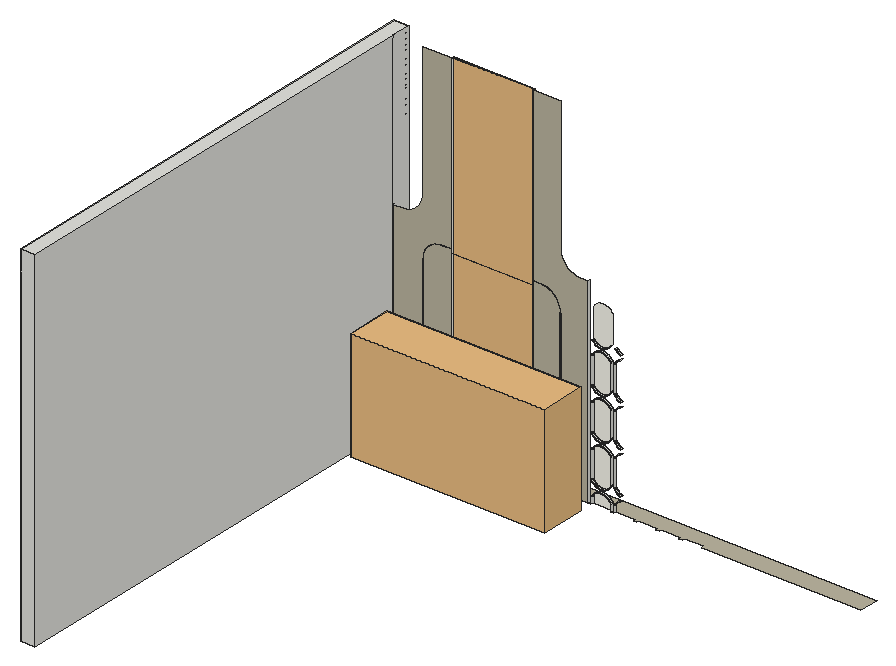
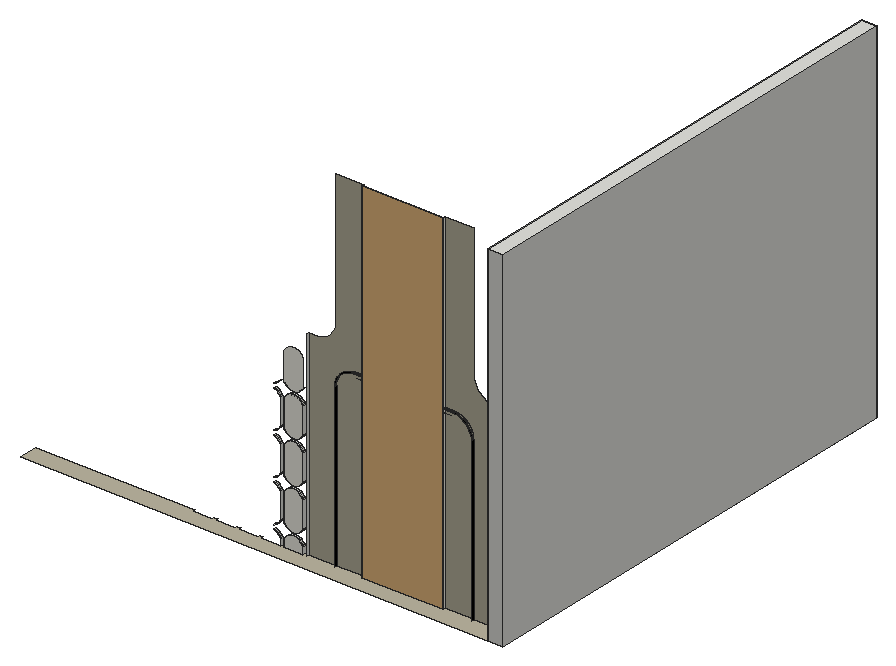
# SketchUp Ruby script. Lengths in inches.
U = 1.inch
M = Sketchup.active_model
def pt(a) = Geom::Point3d.new(a.map { |v| v * U })
def face(e, loops, mat)
  f = e.add_face(loops[0].map { |a| pt(a) })
  loops[1..].each { |l| e.add_face(l.map { |a| pt(a) }).erase! }
  f.material = f.back_material = mat if mat
  f
end
# faces: each face lists its corners as indices into pts; further lists are holes
def faces(e, pts, list, mat = nil) = list.each { |f| face(e, (f[0].is_a?(Array) ? f : [f]).map { |l| l.map { |i| pts[i] } }, mat) }
# xy, xz, yz: faces in a plane at the given z, y or x. An outline is a flat list of corners, or four numbers for a rectangle; further outlines are holes
def ring(l) = l.size == 4 ? [[l[0], l[1]], [l[2], l[1]], [l[2], l[3]], [l[0], l[3]]] : l.each_slice(2).to_a
def flat(e, list, mat, &to3) = list.each { |f| face(e, (f[0].is_a?(Array) ? f : [f]).map { |l| ring(l).map { |u, v| to3.(u, v) } }, mat) }
def xy(e, z, list, mat = nil) = flat(e, list, mat) { |x, y| [x, y, z] }
def xz(e, y, list, mat = nil) = flat(e, list, mat) { |x, z| [x, y, z] }
def yz(e, x, list, mat = nil) = flat(e, list, mat) { |y, z| [x, y, z] }
def lines(e, pts, list) = list.each { |a, b| e.add_line(pt(pts[a]), pt(pts[b])) }
# prism: a flat outline (further loops are holes) pulled along v
def prism(e, loops, v, mat = nil)
  f = face(e, loops, mat); d = Geom::Vector3d.new(v.map { |x| x * U })
  f.pushpull(f.normal.samedirection?(d) ? d.length : -d.length)
end
def box(e, o, s, mat = nil) = prism(e, [[o, [o[0] + s[0], o[1], o[2]], [o[0] + s[0], o[1] + s[1], o[2]], [o[0], o[1] + s[1], o[2]]]], [0, 0, s[2]], mat)
def at(x, y, z, deg = 0) = Geom::Transformation.translation(pt([x, y, z])) * Geom::Transformation.rotation(ORIGIN, Z_AXIS, deg.degrees)
def axes(o, x, y, z) = Geom::Transformation.new([*x, 0, *y, 0, *z, 0, *pt(o).to_a, 1])
def part(name) = M.definitions.add(name)
# library, detail: a bought-in or finely detailed component or shape, given as its bounding box
def library(name, o, s) = part(name).tap { |d| box(d.entities, o, s) }
def detail(e, o, s) = box(e.add_group.entities, o, s)
def put(e, d, t, mat = nil) = e.add_instance(d, t).tap { |i| i.material = mat if mat }
def group(e, t, mat = nil) = e.add_group.tap { |g| g.transformation = t; g.material = mat if mat }.entities
root = M.entities
M.materials.add("Tafisa-Gardenia-or-Gardenia-PM775-4K").color = [246, 245, 235]
M.materials.add("Uniboard-L19-Putty-4K").color = [187, 181, 160]
M.materials.add("[Color M09]").color = [0, 0, 0]
c1 = part("Group196\#1")
p = [[0,0,0],[0,0,-16.77],[-0.04,0,-16.77],[0.28,-54,0],[-0.28,-54,0],[0.28,54,0],
  [0.28,0,0],[-0.28,54,0],[0.04,0,-16.77],[-0.28,0,0],[0,0,-27.14]]
lines(c1.entities,p,[[0,1],[1,2],[3,4],[5,6],[7,5],[1,8],[9,0],[0,6],[8,10],[4,9],[6,3],[2,10],
  [9,7]])
c2 = part("Rectangle Light\#1")
put(c2.entities,c1,at(0,0,0))
c3 = library("Group3\#1",[-12.5,-54,0],[24.96,108,0.24])
c4 = library("Group\#6",[0,0,0],[59.84,14,34])
c5 = part("Group194\#1")
p = [[0,0,0],[0,0,-16.77],[-0.04,0,-16.77],[0.28,-54,0],[-0.28,-54,0],[0.28,54,0],
  [0.28,0,0],[-0.28,54,0],[0.04,0,-16.77],[-0.28,0,0],[0,0,-27.14]]
lines(c5.entities,p,[[0,1],[1,2],[3,4],[5,6],[7,5],[1,8],[9,0],[0,6],[8,10],[4,9],[6,3],[2,10],
  [9,7]])
c6 = part("Rectangle Light")
put(c6.entities,c5,at(0,0,0))
xy(root,6,[[4.5,138,4.5,144,148.5,144,148.5,138,100.62,138,100.62,138.71,100.5,138.71,100.5,138,99.5,138,99.5,138.79,93.5625,138.79,93.5625,138,92.5625,138,92.5625,138.79,86.5,138.79,86.5,138,85.5,138,85.5,138.79,79.5,138.79,79.5,138,78.5,138,78.5,138.79,72.5,138.79,72.5,138,71.5,138,71.5,138.79,65.5,138.79,65.5,138,64.5,138,64.5,138.71,64.38,138.71,64.38,138,56,138,56,138.71,55.76,138.71,55.76,138,47.5,138,47.5,138.79,22.5,138.79,22.5,138,13.74,138,13.74,138.71,13.5,138.71,13.5,138]],"Uniboard-L19-Putty-4K")
xz(root,138,[[4.5,6,13.5,6,13.5,55.5,13.55,56.28,13.7,57.05,13.96,57.8,14.3,58.5,14.74,59.15,15.26,59.74,15.85,60.26,16.5,60.7,17.2,61.04,17.95,61.3,18.72,61.45,19.5,61.5,22.5,61.5,22.5,114,13.5,114,13.5,73.3125,13.45,72.53,13.3,71.76,13.04,71.02,12.7,70.3125,12.26,69.66,11.74,69.07,11.15,68.55,10.5,68.12,9.8,67.77,9.05,67.52,8.28,67.36,7.5,67.3125,4.5,67.3125],[13.74,6,22.5,6,22.5,61.26,19.5,61.26,18.75,61.21,18.01,61.07,17.29,60.83,16.62,60.49,15.99,60.07,15.42,59.58,14.93,59.01,14.51,58.38,14.17,57.71,13.93,56.99,13.79,56.25,13.74,55.5],[47.5,6,55.76,6,55.76,55.5,55.71,56.25,55.57,56.99,55.33,57.71,54.99,58.38,54.57,59.01,54.08,59.58,53.51,60.07,52.88,60.49,52.21,60.83,51.49,61.07,50.75,61.21,50,61.26,47.5,61.26],[56,6,64.38,6,64.38,67.3125,62,67.3125,61.22,67.36,60.45,67.52,59.7,67.77,59,68.12,58.35,68.55,57.76,69.07,57.24,69.66,56.8,70.3125,56.46,71.02,56.2,71.76,56.05,72.53,56,73.3125,56,114,47.5,114,47.5,61.5,50,61.5,50.78,61.45,51.55,61.3,52.3,61.04,53,60.7,53.65,60.26,54.24,59.74,54.76,59.15,55.2,58.5,55.54,57.8,55.8,57.05,55.95,56.28,56,55.5]],"Uniboard-L19-Putty-4K")
xz(root,138.71,[[64.38,6,64.5,67.3125]])
xz(root,138.71,[[13.5,6,13.74,6,13.74,55.5,13.79,56.25,13.93,56.99,14.17,57.71,14.51,58.38,14.93,59.01,15.42,59.58,15.99,60.07,16.62,60.49,17.29,60.83,18.01,61.07,18.75,61.21,19.5,61.26,22.5,61.26,22.5,61.5,19.5,61.5,18.72,61.45,17.95,61.3,17.2,61.04,16.5,60.7,15.85,60.26,15.26,59.74,14.74,59.15,14.3,58.5,13.96,57.8,13.7,57.05,13.55,56.28,13.5,55.5],[55.76,6,56,6,56,55.5,55.95,56.28,55.8,57.05,55.54,57.8,55.2,58.5,54.76,59.15,54.24,59.74,53.65,60.26,53,60.7,52.3,61.04,51.55,61.3,50.78,61.45,50,61.5,47.5,61.5,47.5,61.26,50,61.26,50.75,61.21,51.49,61.07,52.21,60.83,52.88,60.49,53.51,60.07,54.08,59.58,54.57,59.01,54.99,58.38,55.33,57.71,55.57,56.99,55.71,56.25,55.76,55.5]],"[Color M09]")
xz(root,138.79,[[65.5,6,71.5,6,71.5,8,71.36,8.29,71.2,8.56,71.01,8.82,70.79,9.05,70.56,9.26,70.3,9.45,70.03,9.62,69.74,9.75,69.44,9.86,69.13,9.9375,68.82,9.98,68.5,10,68.18,9.98,67.87,9.9375,67.56,9.86,67.26,9.75,66.97,9.62,66.7,9.45,66.44,9.26,66.21,9.05,65.99,8.82,65.8,8.56,65.64,8.29,65.5,8],[68.5,11,68.82,11.02,69.13,11.0625,69.44,11.14,69.74,11.25,70.03,11.38,70.3,11.55,70.56,11.74,70.79,11.95,71.01,12.18,71.2,12.44,71.36,12.71,71.5,13,71.5,21,71.36,21.29,71.2,21.56,71.01,21.82,70.79,22.05,70.56,22.26,70.3,22.45,70.03,22.62,69.74,22.75,69.44,22.86,69.13,22.9375,68.82,22.98,68.5,23,68.18,22.98,67.87,22.9375,67.56,22.86,67.26,22.75,66.97,22.62,66.7,22.45,66.44,22.26,66.21,22.05,65.99,21.82,65.8,21.56,65.64,21.29,65.5,21,65.5,13,65.64,12.71,65.8,12.44,65.99,12.18,66.21,11.95,66.44,11.74,66.7,11.55,66.97,11.38,67.26,11.25,67.56,11.14,67.87,11.0625,68.18,11.02],[68.5,24,68.82,24.02,69.13,24.0625,69.44,24.14,69.74,24.25,70.03,24.38,70.3,24.55,70.56,24.74,70.79,24.95,71.01,25.18,71.2,25.44,71.36,25.71,71.5,26,71.5,34,71.36,34.29,71.2,34.56,71.01,34.82,70.79,35.05,70.56,35.26,70.3,35.45,70.03,35.62,69.74,35.75,69.44,35.86,69.13,35.9375,68.82,35.98,68.5,36,68.18,35.98,67.87,35.9375,67.56,35.86,67.26,35.75,66.97,35.62,66.7,35.45,66.44,35.26,66.21,35.05,65.99,34.82,65.8,34.56,65.64,34.29,65.5,34,65.5,26,65.64,25.71,65.8,25.44,65.99,25.18,66.21,24.95,66.44,24.74,66.7,24.55,66.97,24.38,67.26,24.25,67.56,24.14,67.87,24.0625,68.18,24.02],[68.5,37,68.82,37.02,69.13,37.0625,69.44,37.14,69.74,37.25,70.03,37.38,70.3,37.55,70.56,37.74,70.79,37.95,71.01,38.18,71.2,38.44,71.36,38.71,71.5,39,71.5,47,71.36,47.29,71.2,47.56,71.01,47.82,70.79,48.05,70.56,48.26,70.3,48.45,70.03,48.62,69.74,48.75,69.44,48.86,69.13,48.9375,68.82,48.98,68.5,49,68.18,48.98,67.87,48.9375,67.56,48.86,67.26,48.75,66.97,48.62,66.7,48.45,66.44,48.26,66.21,48.05,65.99,47.82,65.8,47.56,65.64,47.29,65.5,47,65.5,39,65.64,38.71,65.8,38.44,65.99,38.18,66.21,37.95,66.44,37.74,66.7,37.55,66.97,37.38,67.26,37.25,67.56,37.14,67.87,37.0625,68.18,37.02],[68.5,50,68.82,50.02,69.13,50.0625,69.44,50.14,69.74,50.25,70.03,50.38,70.3,50.55,70.56,50.74,70.79,50.95,71.01,51.18,71.2,51.44,71.36,51.71,71.5,52,71.5,60,71.36,60.29,71.2,60.56,71.01,60.82,70.79,61.05,70.56,61.26,70.3,61.45,70.03,61.62,69.74,61.75,69.44,61.86,69.13,61.9375,68.82,61.98,68.5,62,68.18,61.98,67.87,61.9375,67.56,61.86,67.26,61.75,66.97,61.62,66.7,61.45,66.44,61.26,66.21,61.05,65.99,60.82,65.8,60.56,65.64,60.29,65.5,60,65.5,52,65.64,51.71,65.8,51.44,65.99,51.18,66.21,50.95,66.44,50.74,66.7,50.55,66.97,50.38,67.26,50.25,67.56,50.14,67.87,50.0625,68.18,50.02]],"Tafisa-Gardenia-or-Gardenia-PM775-4K")
yz(root,4.5,[[138,6,138,67.3125,138.71,67.3125,138.71,67.55,138,67.55,138,114,144,114,144,6]])
yz(root,13.5,[[138,6,138.71,55.5]],"[Color M09]")
yz(root,13.74,[[138,6,138.71,55.5]],"[Color M09]")
yz(root,47.5,[[138,6,138,61.26,138.71,61.26,138.71,61.5,138,61.5,138,114,138.79,114,138.79,6]],"Tafisa-Gardenia-or-Gardenia-PM775-4K")
yz(root,55.76,[[138,6,138.71,55.5]],"[Color M09]")
yz(root,56,[[138,6,138.71,55.5]],"[Color M09]")
yz(root,64.38,[[138,6,138.71,67.3125]])
yz(root,64.5,[[138,6,138.71,67.3125]])
yz(root,65.5,[[138,6,138.79,8],[138,13,138.79,21],[138,26,138.79,34],[138,39,138.79,47]])
yz(root,71.5,[[138,6,138.79,8],[138,13,138.79,21],[138,26,138.79,34],[138,39,138.79,47]])
yz(root,72.5,[[138,6,138.79,8],[138,13,138.79,21],[138,26,138.79,34],[138,39,138.79,47]])
p = [[65.5,138.79,8],[65.64,138.79,8.29],[65.64,138,8.29],[65.5,138,8],[71.36,138.79,8.29],[71.5,138.79,8],
  [71.5,138,8],[71.36,138,8.29],[72.5,138.79,8],[72.64,138.79,8.29],[72.64,138,8.29],[72.5,138,8],
  [65.8,138.79,8.56],[65.8,138,8.56],[71.2,138.79,8.56],[71.2,138,8.56],[72.8,138.79,8.56],[72.8,138,8.56],
  [65.99,138.79,8.82],[65.99,138,8.82],[71.01,138.79,8.82],[71.01,138,8.82],[72.99,138.79,8.82],[72.99,138,8.82],
  [66.21,138.79,9.05],[66.21,138,9.05],[70.79,138.79,9.05],[70.79,138,9.05],[73.21,138.79,9.05],[73.21,138,9.05],
  [66.44,138.79,9.26],[66.44,138,9.26],[70.56,138.79,9.26],[70.56,138,9.26],[73.44,138.79,9.26],[73.44,138,9.26],
  [66.7,138.79,9.45],[66.7,138,9.45],[70.3,138.79,9.45],[70.3,138,9.45],[73.7,138.79,9.45],[73.7,138,9.45],
  [66.97,138.79,9.62],[66.97,138,9.62],[70.03,138.79,9.62],[70.03,138,9.62],[73.97,138.79,9.62],[73.97,138,9.62],
  [67.26,138.79,9.75],[67.26,138,9.75],[69.74,138.79,9.75],[69.74,138,9.75],[74.26,138.79,9.75],[74.26,138,9.75],
  [67.56,138.79,9.86],[67.56,138,9.86],[69.44,138.79,9.86],[69.44,138,9.86],[74.56,138.79,9.86],[74.56,138,9.86],
  [67.87,138.79,9.9375],[67.87,138,9.9375],[68.18,138.79,9.98],[68.18,138,9.98],[68.82,138.79,9.98],[69.13,138.79,9.9375],
  [69.13,138,9.9375],[68.82,138,9.98],[68.5,138.79,10],[68.5,138,10],[68.18,138.79,11.02],[67.87,138.79,11.0625],
  [67.87,138,11.0625],[68.18,138,11.02],[68.5,138.79,11],[68.5,138,11],[68.82,138.79,11.02],[68.82,138,11.02],
  [69.13,138.79,11.0625],[69.13,138,11.0625],[67.56,138.79,11.14],[67.26,138.79,11.25],[67.26,138,11.25],[67.56,138,11.14],
  [69.44,138.79,11.14],[69.44,138,11.14],[69.74,138.79,11.25],[69.74,138,11.25],[74.56,138.79,11.14],[74.26,138.79,11.25],
  [74.26,138,11.25],[74.56,138,11.14],[66.97,138.79,11.38],[66.97,138,11.38],[70.03,138.79,11.38],[70.03,138,11.38],
  [73.97,138.79,11.38],[73.97,138,11.38],[66.7,138.79,11.55],[66.7,138,11.55],[70.3,138.79,11.55],[70.3,138,11.55],
  [73.7,138.79,11.55],[73.7,138,11.55],[66.44,138.79,11.74],[66.44,138,11.74],[70.56,138.79,11.74],[70.56,138,11.74],
  [73.44,138.79,11.74],[73.44,138,11.74],[66.21,138.79,11.95],[66.21,138,11.95],[70.79,138.79,11.95],[70.79,138,11.95],
  [73.21,138.79,11.95],[73.21,138,11.95],[65.99,138.79,12.18],[65.99,138,12.18],[71.01,138.79,12.18],[71.01,138,12.18],
  [72.99,138.79,12.18],[72.99,138,12.18],[65.8,138.79,12.44],[65.8,138,12.44],[71.2,138.79,12.44],[71.2,138,12.44],
  [72.8,138.79,12.44],[72.8,138,12.44],[65.64,138.79,12.71],[65.64,138,12.71],[71.36,138.79,12.71],[71.36,138,12.71],
  [72.64,138.79,12.71],[72.64,138,12.71],[65.5,138.79,13],[65.5,138,13],[71.5,138.79,13],[71.5,138,13],
  [72.5,138.79,13],[72.5,138,13],[65.5,138.79,21],[65.64,138.79,21.29],[65.64,138,21.29],[65.5,138,21],
  [71.36,138.79,21.29],[71.5,138.79,21],[71.5,138,21],[71.36,138,21.29],[72.5,138.79,21],[72.64,138.79,21.29],
  [72.64,138,21.29],[72.5,138,21],[65.8,138.79,21.56],[65.8,138,21.56],[71.2,138.79,21.56],[71.2,138,21.56],
  [72.8,138.79,21.56],[72.8,138,21.56],[65.99,138.79,21.82],[65.99,138,21.82],[71.01,138.79,21.82],[71.01,138,21.82],
  [72.99,138.79,21.82],[72.99,138,21.82],[66.21,138.79,22.05],[66.21,138,22.05],[70.79,138.79,22.05],[70.79,138,22.05],
  [73.21,138.79,22.05],[73.21,138,22.05],[66.44,138.79,22.26],[66.44,138,22.26],[70.56,138.79,22.26],[70.56,138,22.26],
  [73.44,138.79,22.26],[73.44,138,22.26],[66.7,138.79,22.45],[66.7,138,22.45],[70.3,138.79,22.45],[70.3,138,22.45],
  [73.7,138.79,22.45],[73.7,138,22.45],[66.97,138.79,22.62],[66.97,138,22.62],[70.03,138.79,22.62],[70.03,138,22.62],
  [73.97,138.79,22.62],[73.97,138,22.62],[67.26,138.79,22.75],[67.26,138,22.75],[69.74,138.79,22.75],[69.74,138,22.75],
  [74.26,138.79,22.75],[74.26,138,22.75],[67.56,138.79,22.86],[67.56,138,22.86],[69.44,138.79,22.86],[69.44,138,22.86],
  [74.56,138.79,22.86],[74.56,138,22.86],[67.87,138.79,22.9375],[67.87,138,22.9375],[68.18,138.79,22.98],[68.18,138,22.98],
  [68.82,138.79,22.98],[69.13,138.79,22.9375],[69.13,138,22.9375],[68.82,138,22.98],[68.5,138.79,23],[68.5,138,23],
  [68.18,138.79,24.02],[67.87,138.79,24.0625],[67.87,138,24.0625],[68.18,138,24.02],[68.5,138.79,24],[68.5,138,24],
  [68.82,138.79,24.02],[68.82,138,24.02],[69.13,138.79,24.0625],[69.13,138,24.0625],[67.56,138.79,24.14],[67.26,138.79,24.25],
  [67.26,138,24.25],[67.56,138,24.14],[69.44,138.79,24.14],[69.44,138,24.14],[69.74,138.79,24.25],[69.74,138,24.25],
  [74.56,138.79,24.14],[74.26,138.79,24.25],[74.26,138,24.25],[74.56,138,24.14],[66.97,138.79,24.38],[66.97,138,24.38],
  [70.03,138.79,24.38],[70.03,138,24.38],[73.97,138.79,24.38],[73.97,138,24.38],[66.7,138.79,24.55],[66.7,138,24.55],
  [70.3,138.79,24.55],[70.3,138,24.55],[73.7,138.79,24.55],[73.7,138,24.55],[66.44,138.79,24.74],[66.44,138,24.74],
  [70.56,138.79,24.74],[70.56,138,24.74],[73.44,138.79,24.74],[73.44,138,24.74],[66.21,138.79,24.95],[66.21,138,24.95],
  [70.79,138.79,24.95],[70.79,138,24.95],[73.21,138.79,24.95],[73.21,138,24.95],[65.99,138.79,25.18],[65.99,138,25.18],
  [71.01,138.79,25.18],[71.01,138,25.18],[72.99,138.79,25.18],[72.99,138,25.18],[65.8,138.79,25.44],[65.8,138,25.44],
  [71.2,138.79,25.44],[71.2,138,25.44],[72.8,138.79,25.44],[72.8,138,25.44],[65.64,138.79,25.71],[65.64,138,25.71],
  [71.36,138.79,25.71],[71.36,138,25.71],[72.64,138.79,25.71],[72.64,138,25.71],[65.5,138.79,26],[65.5,138,26],
  [71.5,138.79,26],[71.5,138,26],[72.5,138.79,26],[72.5,138,26],[65.5,138.79,34],[65.64,138.79,34.29],
  [65.64,138,34.29],[65.5,138,34],[71.36,138.79,34.29],[71.5,138.79,34],[71.5,138,34],[71.36,138,34.29],
  [72.5,138.79,34],[72.64,138.79,34.29],[72.64,138,34.29],[72.5,138,34],[65.8,138.79,34.56],[65.8,138,34.56],
  [71.2,138.79,34.56],[71.2,138,34.56],[72.8,138.79,34.56],[72.8,138,34.56],[65.99,138.79,34.82],[65.99,138,34.82],
  [71.01,138.79,34.82],[71.01,138,34.82],[72.99,138.79,34.82],[72.99,138,34.82],[66.21,138.79,35.05],[66.21,138,35.05],
  [70.79,138.79,35.05],[70.79,138,35.05],[73.21,138.79,35.05],[73.21,138,35.05],[66.44,138.79,35.26],[66.44,138,35.26],
  [70.56,138.79,35.26],[70.56,138,35.26],[73.44,138.79,35.26],[73.44,138,35.26],[66.7,138.79,35.45],[66.7,138,35.45],
  [70.3,138.79,35.45],[70.3,138,35.45],[73.7,138.79,35.45],[73.7,138,35.45],[66.97,138.79,35.62],[66.97,138,35.62],
  [70.03,138.79,35.62],[70.03,138,35.62],[73.97,138.79,35.62],[73.97,138,35.62],[67.26,138.79,35.75],[67.26,138,35.75],
  [69.74,138.79,35.75],[69.74,138,35.75],[74.26,138.79,35.75],[74.26,138,35.75],[67.56,138.79,35.86],[67.56,138,35.86],
  [69.44,138.79,35.86],[69.44,138,35.86],[74.56,138.79,35.86],[74.56,138,35.86],[67.87,138.79,35.9375],[67.87,138,35.9375],
  [68.18,138.79,35.98],[68.18,138,35.98],[68.82,138.79,35.98],[69.13,138.79,35.9375],[69.13,138,35.9375],[68.82,138,35.98],
  [68.5,138.79,36],[68.5,138,36],[68.18,138.79,37.02],[67.87,138.79,37.0625],[67.87,138,37.0625],[68.18,138,37.02],
  [68.5,138.79,37],[68.5,138,37],[68.82,138.79,37.02],[68.82,138,37.02],[69.13,138.79,37.0625],[69.13,138,37.0625],
  [67.56,138.79,37.14],[67.26,138.79,37.25],[67.26,138,37.25],[67.56,138,37.14],[69.44,138.79,37.14],[69.44,138,37.14],
  [69.74,138.79,37.25],[69.74,138,37.25],[74.56,138.79,37.14],[74.26,138.79,37.25],[74.26,138,37.25],[74.56,138,37.14],
  [66.97,138.79,37.38],[66.97,138,37.38],[70.03,138.79,37.38],[70.03,138,37.38],[73.97,138.79,37.38],[73.97,138,37.38],
  [66.7,138.79,37.55],[66.7,138,37.55],[70.3,138.79,37.55],[70.3,138,37.55],[73.7,138.79,37.55],[73.7,138,37.55],
  [66.44,138.79,37.74],[66.44,138,37.74],[70.56,138.79,37.74],[70.56,138,37.74],[73.44,138.79,37.74],[73.44,138,37.74],
  [66.21,138.79,37.95],[66.21,138,37.95],[70.79,138.79,37.95],[70.79,138,37.95],[73.21,138.79,37.95],[73.21,138,37.95],
  [65.99,138.79,38.18],[65.99,138,38.18],[71.01,138.79,38.18],[71.01,138,38.18],[72.99,138.79,38.18],[72.99,138,38.18],
  [65.8,138.79,38.44],[65.8,138,38.44],[71.2,138.79,38.44],[71.2,138,38.44],[72.8,138.79,38.44],[72.8,138,38.44],
  [65.64,138.79,38.71],[65.64,138,38.71],[71.36,138.79,38.71],[71.36,138,38.71],[72.64,138.79,38.71],[72.64,138,38.71],
  [65.5,138.79,39],[65.5,138,39],[71.5,138.79,39],[71.5,138,39],[72.5,138.79,39],[72.5,138,39],
  [65.5,138.79,47],[65.64,138.79,47.29],[65.64,138,47.29],[65.5,138,47],[71.36,138.79,47.29],[71.5,138.79,47],
  [71.5,138,47],[71.36,138,47.29],[72.5,138.79,47],[72.64,138.79,47.29],[72.64,138,47.29],[72.5,138,47],
  [65.8,138.79,47.56],[65.8,138,47.56],[71.2,138.79,47.56],[71.2,138,47.56],[72.8,138.79,47.56],[72.8,138,47.56],
  [65.99,138.79,47.82],[65.99,138,47.82],[71.01,138.79,47.82],[71.01,138,47.82],[72.99,138.79,47.82],[72.99,138,47.82],
  [66.21,138.79,48.05],[66.21,138,48.05],[70.79,138.79,48.05],[70.79,138,48.05],[73.21,138.79,48.05],[73.21,138,48.05],
  [66.44,138.79,48.26],[66.44,138,48.26],[70.56,138.79,48.26],[70.56,138,48.26],[73.44,138.79,48.26],[73.44,138,48.26],
  [66.7,138.79,48.45],[66.7,138,48.45],[70.3,138.79,48.45],[70.3,138,48.45],[73.7,138.79,48.45],[73.7,138,48.45],
  [66.97,138.79,48.62],[66.97,138,48.62],[70.03,138.79,48.62],[70.03,138,48.62],[73.97,138.79,48.62],[73.97,138,48.62],
  [67.26,138.79,48.75],[67.26,138,48.75],[69.74,138.79,48.75],[69.74,138,48.75],[74.26,138.79,48.75],[74.26,138,48.75],
  [67.56,138.79,48.86],[67.56,138,48.86],[69.44,138.79,48.86],[69.44,138,48.86],[74.56,138.79,48.86],[74.56,138,48.86],
  [67.87,138.79,48.9375],[67.87,138,48.9375],[68.18,138.79,48.98],[68.18,138,48.98],[68.82,138.79,48.98],[69.13,138.79,48.9375],
  [69.13,138,48.9375],[68.82,138,48.98],[68.5,138.79,49],[68.5,138,49],[68.18,138.79,50.02],[67.87,138.79,50.0625],
  [67.87,138,50.0625],[68.18,138,50.02],[68.5,138.79,50],[68.5,138,50],[68.82,138.79,50.02],[68.82,138,50.02],
  [69.13,138.79,50.0625],[69.13,138,50.0625],[67.56,138.79,50.14],[67.26,138.79,50.25],[67.26,138,50.25],[67.56,138,50.14],
  [69.44,138.79,50.14],[69.44,138,50.14],[69.74,138.79,50.25],[69.74,138,50.25],[74.56,138.79,50.14],[74.26,138.79,50.25],
  [74.26,138,50.25],[74.56,138,50.14],[66.97,138.79,50.38],[66.97,138,50.38],[70.03,138.79,50.38],[70.03,138,50.38],
  [73.97,138.79,50.38],[73.97,138,50.38],[66.7,138.79,50.55],[66.7,138,50.55],[70.3,138.79,50.55],[70.3,138,50.55],
  [73.7,138.79,50.55],[73.7,138,50.55],[66.44,138.79,50.74],[66.44,138,50.74],[70.56,138.79,50.74],[70.56,138,50.74],
  [73.44,138.79,50.74],[73.44,138,50.74],[66.21,138.79,50.95],[66.21,138,50.95],[70.79,138.79,50.95],[70.79,138,50.95],
  [73.21,138.79,50.95],[73.21,138,50.95],[65.99,138.79,51.18],[65.99,138,51.18],[71.01,138.79,51.18],[71.01,138,51.18],
  [72.99,138.79,51.18],[72.99,138,51.18],[65.8,138.79,51.44],[65.8,138,51.44],[71.2,138.79,51.44],[71.2,138,51.44],
  [72.8,138.79,51.44],[72.8,138,51.44]]
faces(root,p,[[0,1,2,3],[4,5,6,7],[8,9,10,11],[1,12,13,2],[14,4,7,15],[9,16,17,10],[12,18,19,13],[20,14,15,21],
  [16,22,23,17],[18,24,25,19],[26,20,21,27],[22,28,29,23],[24,30,31,25],[32,26,27,33],[28,34,35,29],[30,36,37,31],
  [38,32,33,39],[34,40,41,35],[36,42,43,37],[44,38,39,45],[40,46,47,41],[42,48,49,43],[50,44,45,51],[46,52,53,47],
  [48,54,55,49],[56,50,51,57],[52,58,59,53],[54,60,61,55],[60,62,63,61],[64,65,66,67],[65,56,57,66],[62,68,69,63],
  [68,64,67,69],[70,71,72,73],[74,70,73,75],[76,74,75,77],[78,76,77,79],[80,81,82,83],[71,80,83,72],[84,78,79,85],
  [86,84,85,87],[88,89,90,91],[81,92,93,82],[94,86,87,95],[89,96,97,90],[92,98,99,93],[100,94,95,101],[96,102,103,97],
  [98,104,105,99],[106,100,101,107],[102,108,109,103],[104,110,111,105],[112,106,107,113],[108,114,115,109],[110,116,117,111],[118,112,113,119],
  [114,120,121,115],[116,122,123,117],[124,118,119,125],[120,126,127,121],[122,128,129,123],[130,124,125,131],[126,132,133,127],[128,134,135,129],
  [136,130,131,137],[132,138,139,133],[140,141,142,143],[144,145,146,147],[148,149,150,151],[141,152,153,142],[154,144,147,155],[149,156,157,150],
  [152,158,159,153],[160,154,155,161],[156,162,163,157],[158,164,165,159],[166,160,161,167],[162,168,169,163],[164,170,171,165],[172,166,167,173],
  [168,174,175,169],[170,176,177,171],[178,172,173,179],[174,180,181,175],[176,182,183,177],[184,178,179,185],[180,186,187,181],[182,188,189,183],
  [190,184,185,191],[186,192,193,187],[188,194,195,189],[196,190,191,197],[192,198,199,193],[194,200,201,195],[200,202,203,201],[204,205,206,207],
  [205,196,197,206],[202,208,209,203],[208,204,207,209],[210,211,212,213],[214,210,213,215],[216,214,215,217],[218,216,217,219],[220,221,222,223],
  [211,220,223,212],[224,218,219,225],[226,224,225,227],[228,229,230,231],[221,232,233,222],[234,226,227,235],[229,236,237,230],[232,238,239,233],
  [240,234,235,241],[236,242,243,237],[238,244,245,239],[246,240,241,247],[242,248,249,243],[244,250,251,245],[252,246,247,253],[248,254,255,249],
  [250,256,257,251],[258,252,253,259],[254,260,261,255],[256,262,263,257],[264,258,259,265],[260,266,267,261],[262,268,269,263],[270,264,265,271],
  [266,272,273,267],[268,274,275,269],[276,270,271,277],[272,278,279,273],[280,281,282,283],[284,285,286,287],[288,289,290,291],[281,292,293,282],
  [294,284,287,295],[289,296,297,290],[292,298,299,293],[300,294,295,301],[296,302,303,297],[298,304,305,299],[306,300,301,307],[302,308,309,303],
  [304,310,311,305],[312,306,307,313],[308,314,315,309],[310,316,317,311],[318,312,313,319],[314,320,321,315],[316,322,323,317],[324,318,319,325],
  [320,326,327,321],[322,328,329,323],[330,324,325,331],[326,332,333,327],[328,334,335,329],[336,330,331,337],[332,338,339,333],[334,340,341,335],
  [340,342,343,341],[344,345,346,347],[345,336,337,346],[342,348,349,343],[348,344,347,349],[350,351,352,353],[354,350,353,355],[356,354,355,357],
  [358,356,357,359],[360,361,362,363],[351,360,363,352],[364,358,359,365],[366,364,365,367],[368,369,370,371],[361,372,373,362],[374,366,367,375],
  [369,376,377,370],[372,378,379,373],[380,374,375,381],[376,382,383,377],[378,384,385,379],[386,380,381,387],[382,388,389,383],[384,390,391,385],
  [392,386,387,393],[388,394,395,389],[390,396,397,391],[398,392,393,399],[394,400,401,395],[396,402,403,397],[404,398,399,405],[400,406,407,401],
  [402,408,409,403],[410,404,405,411],[406,412,413,407],[408,414,415,409],[416,410,411,417],[412,418,419,413],[420,421,422,423],[424,425,426,427],
  [428,429,430,431],[421,432,433,422],[434,424,427,435],[429,436,437,430],[432,438,439,433],[440,434,435,441],[436,442,443,437],[438,444,445,439],
  [446,440,441,447],[442,448,449,443],[444,450,451,445],[452,446,447,453],[448,454,455,449],[450,456,457,451],[458,452,453,459],[454,460,461,455],
  [456,462,463,457],[464,458,459,465],[460,466,467,461],[462,468,469,463],[470,464,465,471],[466,472,473,467],[468,474,475,469],[476,470,471,477],
  [472,478,479,473],[474,480,481,475],[480,482,483,481],[484,485,486,487],[485,476,477,486],[482,488,489,483],[488,484,487,489],[490,491,492,493],
  [494,490,493,495],[496,494,495,497],[498,496,497,499],[500,501,502,503],[491,500,503,492],[504,498,499,505],[506,504,505,507],[508,509,510,511],
  [501,512,513,502],[514,506,507,515],[509,516,517,510],[512,518,519,513],[520,514,515,521],[516,522,523,517],[518,524,525,519],[526,520,521,527],
  [522,528,529,523],[524,530,531,525],[532,526,527,533],[528,534,535,529],[530,536,537,531],[538,532,533,539],[534,540,541,535],[536,542,543,537],
  [544,538,539,545],[540,546,547,541]])
g1 = group(root,at(0,0,5.88))
box(g1,[0,0,0],[4.5,144,108.12])
g2 = group(root,at(22.5,138,6))
yz(g2,0,[[0,0,0.79,0,0.79,108,0,108,0,55.5,0.71,55.5,0.71,55.26,0,55.26]],"Tafisa-Gardenia-or-Gardenia-PM775-4K")
put(root,c2,axes([47.49,138.28,60],[0,-1,0],[0,0,-1],[1,0,0]))
put(root,c3,axes([35,138.79,60],[1,0,0],[0,0,1],[0,-1,0]),"Tafisa-Gardenia-or-Gardenia-PM775-4K")
put(root,c4,at(5.48,120.25,5.88),"Tafisa-Gardenia-or-Gardenia-PM775-4K")
put(root,c6,axes([22.51,138.28,60],[0,-1,0],[0,0,-1],[-1,0,0]))
